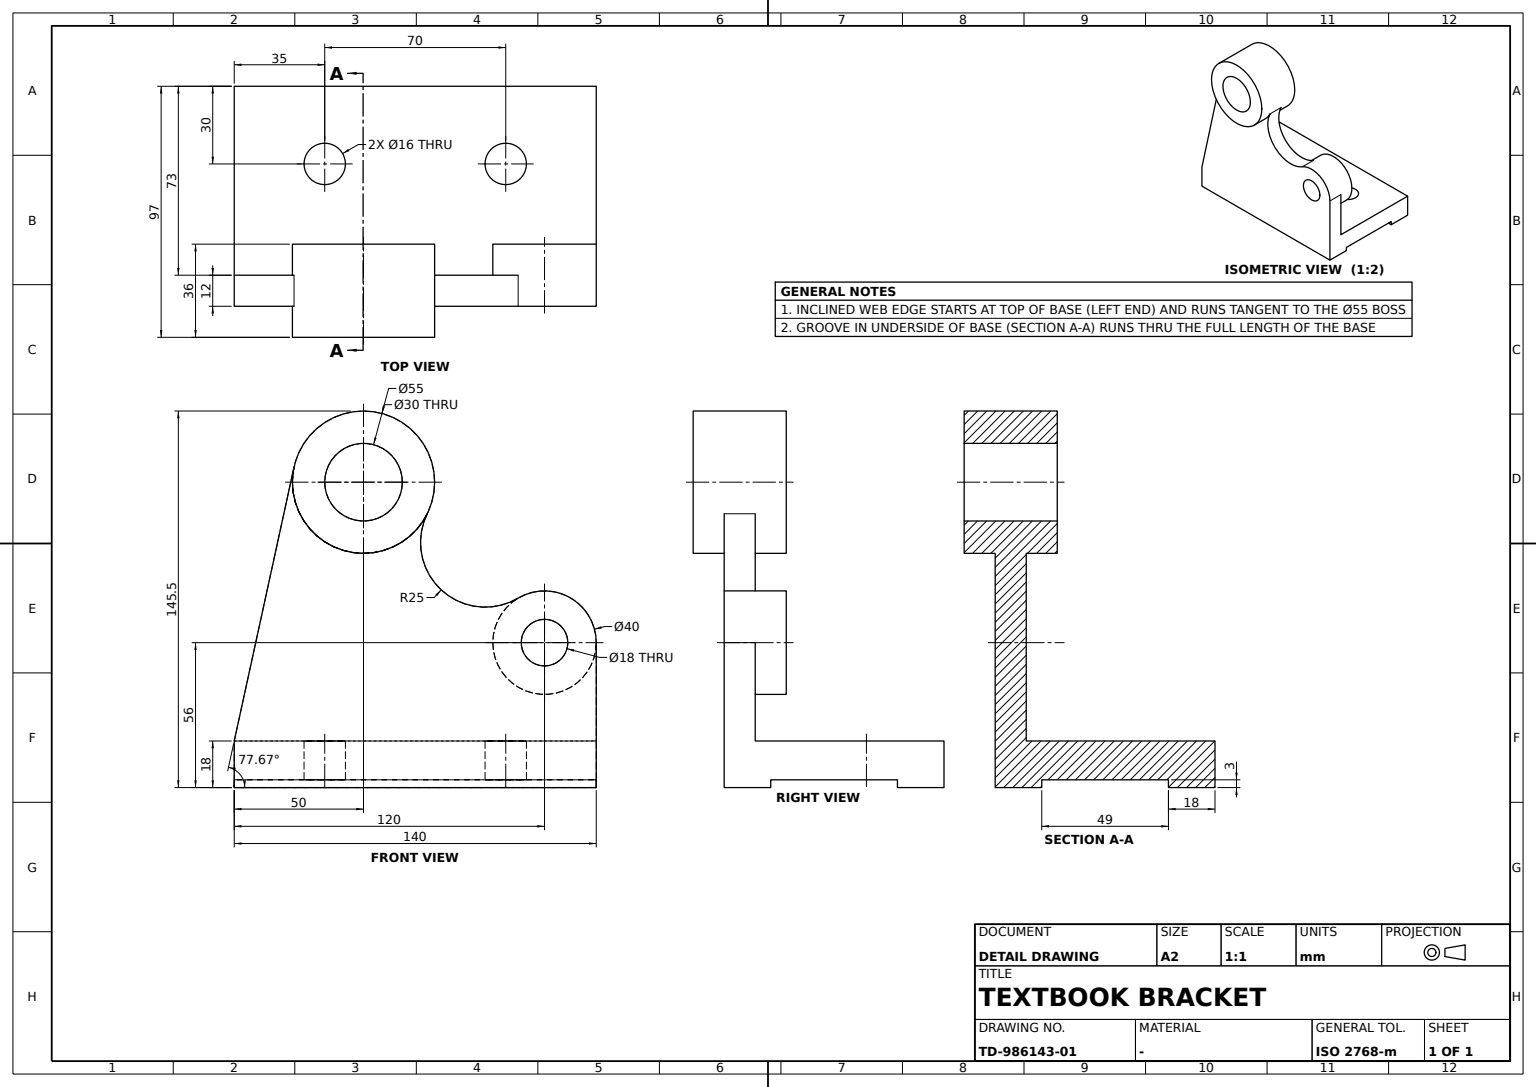
ISO-10303-21;
HEADER;
FILE_DESCRIPTION((''),'2;1');
FILE_NAME('','',(''),(''),'','','');
FILE_SCHEMA(('AUTOMOTIVE_DESIGN'));
ENDSEC;
DATA;
#1=APPLICATION_CONTEXT('');
#2=PRODUCT_CONTEXT('',#1,'mechanical');
#3=PRODUCT('','','',(#2));
#4=PRODUCT_DEFINITION_FORMATION('','',#3);
#5=PRODUCT_DEFINITION_CONTEXT('',#1,'design');
#6=PRODUCT_DEFINITION('','',#4,#5);
#7=PRODUCT_DEFINITION_SHAPE('','',#6);
#8=(LENGTH_UNIT()NAMED_UNIT(*)SI_UNIT(.MILLI.,.METRE.));
#9=(NAMED_UNIT(*)PLANE_ANGLE_UNIT()SI_UNIT($,.RADIAN.));
#10=(NAMED_UNIT(*)SI_UNIT($,.STERADIAN.)SOLID_ANGLE_UNIT());
#11=UNCERTAINTY_MEASURE_WITH_UNIT(LENGTH_MEASURE(1.E-05),#8,'distance_accuracy_value','');
#12=(GEOMETRIC_REPRESENTATION_CONTEXT(3)GLOBAL_UNCERTAINTY_ASSIGNED_CONTEXT((#11))GLOBAL_UNIT_ASSIGNED_CONTEXT((#8,#9,#10))REPRESENTATION_CONTEXT('',''));
#13=CARTESIAN_POINT('',(43.,12.5,0.));
#14=VERTEX_POINT('',#13);
#15=CARTESIAN_POINT('',(43.,12.5,-15.));
#16=VERTEX_POINT('',#15);
#17=CARTESIAN_POINT('',(43.,12.5,-35.));
#18=DIRECTION('',(0.,0.,-1.));
#19=VECTOR('',#18,1000.);
#20=LINE('',#17,#19);
#21=EDGE_CURVE('',#14,#16,#20,.T.);
#22=ORIENTED_EDGE('',*,*,#21,.F.);
#23=CARTESIAN_POINT('',(27.,12.5,0.));
#24=VERTEX_POINT('',#23);
#25=CARTESIAN_POINT('',(35.,12.5,0.));
#26=DIRECTION('',(0.,0.,1.));
#27=DIRECTION('',(1.,0.,0.));
#28=AXIS2_PLACEMENT_3D('',#25,#26,#27);
#29=CIRCLE('',#28,8.);
#30=EDGE_CURVE('',#14,#24,#29,.T.);
#31=ORIENTED_EDGE('',*,*,#30,.T.);
#32=CARTESIAN_POINT('',(27.,12.5,-15.));
#33=VERTEX_POINT('',#32);
#34=CARTESIAN_POINT('',(27.,12.5,-35.));
#35=LINE('',#34,#19);
#36=EDGE_CURVE('',#24,#33,#35,.T.);
#37=ORIENTED_EDGE('',*,*,#36,.T.);
#38=CARTESIAN_POINT('',(35.,12.5,-15.));
#39=DIRECTION('',(0.,1.,0.));
#40=AXIS2_PLACEMENT_3D('',#38,#18,#39);
#41=CIRCLE('',#40,8.);
#42=EDGE_CURVE('',#33,#16,#41,.T.);
#43=ORIENTED_EDGE('',*,*,#42,.T.);
#44=EDGE_LOOP('',(#22,#31,#37,#43));
#45=FACE_OUTER_BOUND('',#44,.T.);
#46=CARTESIAN_POINT('',(35.,12.5,-35.));
#47=AXIS2_PLACEMENT_3D('',#46,#18,#27);
#48=CYLINDRICAL_SURFACE('',#47,8.);
#49=ADVANCED_FACE('',(#45),#48,.F.);
#50=CARTESIAN_POINT('',(70.,-30.5,38.));
#51=VERTEX_POINT('',#50);
#52=CARTESIAN_POINT('',(70.,-18.5,38.));
#53=VERTEX_POINT('',#52);
#54=CARTESIAN_POINT('',(70.,-39.5,38.));
#55=VECTOR('',#39,1000.);
#56=LINE('',#54,#55);
#57=EDGE_CURVE('',#51,#53,#56,.T.);
#58=ORIENTED_EDGE('',*,*,#57,.F.);
#59=CARTESIAN_POINT('',(30.,-30.5,38.));
#60=VERTEX_POINT('',#59);
#61=CARTESIAN_POINT('',(50.,-30.5,38.));
#62=AXIS2_PLACEMENT_3D('',#61,#39,#27);
#63=CIRCLE('',#62,20.);
#64=EDGE_CURVE('',#51,#60,#63,.T.);
#65=ORIENTED_EDGE('',*,*,#64,.T.);
#66=CARTESIAN_POINT('',(30.,-18.5,38.));
#67=VERTEX_POINT('',#66);
#68=CARTESIAN_POINT('',(30.,-39.5,38.));
#69=LINE('',#68,#55);
#70=EDGE_CURVE('',#60,#67,#69,.T.);
#71=ORIENTED_EDGE('',*,*,#70,.T.);
#72=CARTESIAN_POINT('',(50.,-18.5,38.));
#73=DIRECTION('',(0.,-1.,0.));
#74=AXIS2_PLACEMENT_3D('',#72,#73,#27);
#75=CIRCLE('',#74,20.);
#76=EDGE_CURVE('',#67,#53,#75,.T.);
#77=ORIENTED_EDGE('',*,*,#76,.T.);
#78=EDGE_LOOP('',(#58,#65,#71,#77));
#79=FACE_OUTER_BOUND('',#78,.T.);
#80=CYLINDRICAL_SURFACE('',#62,20.);
#81=ADVANCED_FACE('',(#79),#80,.T.);
#82=CARTESIAN_POINT('',(39.8001548126,-30.5,55.2035798063));
#83=VERTEX_POINT('',#82);
#84=EDGE_CURVE('',#60,#83,#63,.T.);
#85=ORIENTED_EDGE('',*,*,#84,.F.);
#86=ORIENTED_EDGE('',*,*,#64,.F.);
#87=CARTESIAN_POINT('',(70.,-30.5,0.));
#88=VERTEX_POINT('',#87);
#89=CARTESIAN_POINT('',(70.,-30.5,19.));
#90=VECTOR('',#26,1000.);
#91=LINE('',#89,#90);
#92=EDGE_CURVE('',#88,#51,#91,.T.);
#93=ORIENTED_EDGE('',*,*,#92,.F.);
#94=CARTESIAN_POINT('',(-70.,-30.5,0.));
#95=VERTEX_POINT('',#94);
#96=CARTESIAN_POINT('',(0.,-30.5,0.));
#97=VECTOR('',#27,1000.);
#98=LINE('',#96,#97);
#99=EDGE_CURVE('',#95,#88,#98,.T.);
#100=ORIENTED_EDGE('',*,*,#99,.F.);
#101=CARTESIAN_POINT('',(-46.8660884819,-30.5,105.8705442409));
#102=VERTEX_POINT('',#101);
#103=CARTESIAN_POINT('',(-58.4330442409,-30.5,52.9352721205));
#104=DIRECTION('',(-0.213474336,0.,-0.9769486721));
#105=VECTOR('',#104,1000.);
#106=LINE('',#103,#105);
#107=EDGE_CURVE('',#102,#95,#106,.T.);
#108=ORIENTED_EDGE('',*,*,#107,.F.);
#109=CARTESIAN_POINT('',(-47.5,-30.5,100.));
#110=VERTEX_POINT('',#109);
#111=CARTESIAN_POINT('',(-20.,-30.5,100.));
#112=AXIS2_PLACEMENT_3D('',#111,#39,#27);
#113=CIRCLE('',#112,27.5);
#114=EDGE_CURVE('',#110,#102,#113,.T.);
#115=ORIENTED_EDGE('',*,*,#114,.F.);
#116=CARTESIAN_POINT('',(4.6454205529,-30.5,87.7994571527));
#117=VERTEX_POINT('',#116);
#118=EDGE_CURVE('',#117,#110,#113,.T.);
#119=ORIENTED_EDGE('',*,*,#118,.F.);
#120=CARTESIAN_POINT('',(27.0503483283,-30.5,76.7080545643));
#121=AXIS2_PLACEMENT_3D('',#120,#39,#27);
#122=CIRCLE('',#121,25.);
#123=EDGE_CURVE('',#83,#117,#122,.T.);
#124=ORIENTED_EDGE('',*,*,#123,.F.);
#125=EDGE_LOOP('',(#85,#86,#93,#100,#108,#115,#119,#124));
#126=FACE_OUTER_BOUND('',#125,.T.);
#127=AXIS2_PLACEMENT_3D('',#96,#73,#27);
#128=PLANE('',#127);
#129=ADVANCED_FACE('',(#126),#128,.F.);
#130=CARTESIAN_POINT('',(-27.,12.5,0.));
#131=VERTEX_POINT('',#130);
#132=CARTESIAN_POINT('',(-27.,12.5,-15.));
#133=VERTEX_POINT('',#132);
#134=CARTESIAN_POINT('',(-27.,12.5,-35.));
#135=LINE('',#134,#19);
#136=EDGE_CURVE('',#131,#133,#135,.T.);
#137=ORIENTED_EDGE('',*,*,#136,.T.);
#138=CARTESIAN_POINT('',(-43.,12.5,-15.));
#139=VERTEX_POINT('',#138);
#140=CARTESIAN_POINT('',(-35.,12.5,-15.));
#141=AXIS2_PLACEMENT_3D('',#140,#18,#39);
#142=CIRCLE('',#141,8.);
#143=EDGE_CURVE('',#133,#139,#142,.T.);
#144=ORIENTED_EDGE('',*,*,#143,.T.);
#145=CARTESIAN_POINT('',(-43.,12.5,0.));
#146=VERTEX_POINT('',#145);
#147=CARTESIAN_POINT('',(-43.,12.5,-35.));
#148=LINE('',#147,#19);
#149=EDGE_CURVE('',#146,#139,#148,.T.);
#150=ORIENTED_EDGE('',*,*,#149,.F.);
#151=CARTESIAN_POINT('',(-35.,12.5,0.));
#152=AXIS2_PLACEMENT_3D('',#151,#26,#27);
#153=CIRCLE('',#152,8.);
#154=EDGE_CURVE('',#146,#131,#153,.T.);
#155=ORIENTED_EDGE('',*,*,#154,.T.);
#156=EDGE_LOOP('',(#137,#144,#150,#155));
#157=FACE_OUTER_BOUND('',#156,.T.);
#158=CARTESIAN_POINT('',(-35.,12.5,-35.));
#159=AXIS2_PLACEMENT_3D('',#158,#18,#27);
#160=CYLINDRICAL_SURFACE('',#159,8.);
#161=ADVANCED_FACE('',(#157),#160,.F.);
#162=CARTESIAN_POINT('',(59.,-18.5,38.));
#163=VERTEX_POINT('',#162);
#164=CARTESIAN_POINT('',(41.,-18.5,38.));
#165=VERTEX_POINT('',#164);
#166=DIRECTION('',(-1.,0.,0.));
#167=AXIS2_PLACEMENT_3D('',#72,#39,#166);
#168=CIRCLE('',#167,9.);
#169=EDGE_CURVE('',#163,#165,#168,.T.);
#170=ORIENTED_EDGE('',*,*,#169,.T.);
#171=CARTESIAN_POINT('',(41.,-42.5,38.));
#172=VERTEX_POINT('',#171);
#173=CARTESIAN_POINT('',(41.,-30.5,38.));
#174=VECTOR('',#73,1000.);
#175=LINE('',#173,#174);
#176=EDGE_CURVE('',#165,#172,#175,.T.);
#177=ORIENTED_EDGE('',*,*,#176,.T.);
#178=CARTESIAN_POINT('',(59.,-42.5,38.));
#179=VERTEX_POINT('',#178);
#180=CARTESIAN_POINT('',(50.,-42.5,38.));
#181=AXIS2_PLACEMENT_3D('',#180,#39,#166);
#182=CIRCLE('',#181,9.);
#183=EDGE_CURVE('',#179,#172,#182,.T.);
#184=ORIENTED_EDGE('',*,*,#183,.F.);
#185=CARTESIAN_POINT('',(59.,-30.5,38.));
#186=LINE('',#185,#174);
#187=EDGE_CURVE('',#163,#179,#186,.T.);
#188=ORIENTED_EDGE('',*,*,#187,.F.);
#189=EDGE_LOOP('',(#170,#177,#184,#188));
#190=FACE_OUTER_BOUND('',#189,.T.);
#191=AXIS2_PLACEMENT_3D('',#61,#73,#166);
#192=CYLINDRICAL_SURFACE('',#191,9.);
#193=ADVANCED_FACE('',(#190),#192,.F.);
#194=CARTESIAN_POINT('',(39.8001548126,-42.5,55.2035798063));
#195=VERTEX_POINT('',#194);
#196=CARTESIAN_POINT('',(4.6454205529,-42.5,87.7994571527));
#197=VERTEX_POINT('',#196);
#198=CARTESIAN_POINT('',(27.0503483283,-42.5,76.7080545643));
#199=AXIS2_PLACEMENT_3D('',#198,#39,#27);
#200=CIRCLE('',#199,25.);
#201=EDGE_CURVE('',#195,#197,#200,.T.);
#202=ORIENTED_EDGE('',*,*,#201,.F.);
#203=CARTESIAN_POINT('',(39.8001548126,-39.5,55.2035798063));
#204=LINE('',#203,#55);
#205=EDGE_CURVE('',#195,#83,#204,.T.);
#206=ORIENTED_EDGE('',*,*,#205,.T.);
#207=ORIENTED_EDGE('',*,*,#123,.T.);
#208=CARTESIAN_POINT('',(4.6454205529,-36.5,87.7994571527));
#209=LINE('',#208,#55);
#210=EDGE_CURVE('',#197,#117,#209,.T.);
#211=ORIENTED_EDGE('',*,*,#210,.F.);
#212=EDGE_LOOP('',(#202,#206,#207,#211));
#213=FACE_OUTER_BOUND('',#212,.T.);
#214=CARTESIAN_POINT('',(27.0503483283,-36.5,76.7080545643));
#215=AXIS2_PLACEMENT_3D('',#214,#39,#27);
#216=CYLINDRICAL_SURFACE('',#215,25.);
#217=ADVANCED_FACE('',(#213),#216,.F.);
#218=CARTESIAN_POINT('',(-70.,24.5,-18.));
#219=VERTEX_POINT('',#218);
#220=CARTESIAN_POINT('',(70.,24.5,-18.));
#221=VERTEX_POINT('',#220);
#222=CARTESIAN_POINT('',(0.,24.5,-18.));
#223=LINE('',#222,#97);
#224=EDGE_CURVE('',#219,#221,#223,.T.);
#225=ORIENTED_EDGE('',*,*,#224,.F.);
#226=CARTESIAN_POINT('',(-70.,42.5,-18.));
#227=VERTEX_POINT('',#226);
#228=CARTESIAN_POINT('',(-70.,33.5,-18.));
#229=LINE('',#228,#55);
#230=EDGE_CURVE('',#219,#227,#229,.T.);
#231=ORIENTED_EDGE('',*,*,#230,.T.);
#232=CARTESIAN_POINT('',(70.,42.5,-18.));
#233=VERTEX_POINT('',#232);
#234=CARTESIAN_POINT('',(0.,42.5,-18.));
#235=LINE('',#234,#97);
#236=EDGE_CURVE('',#227,#233,#235,.T.);
#237=ORIENTED_EDGE('',*,*,#236,.T.);
#238=CARTESIAN_POINT('',(70.,33.5,-18.));
#239=LINE('',#238,#55);
#240=EDGE_CURVE('',#221,#233,#239,.T.);
#241=ORIENTED_EDGE('',*,*,#240,.F.);
#242=EDGE_LOOP('',(#225,#231,#237,#241));
#243=FACE_OUTER_BOUND('',#242,.T.);
#244=CARTESIAN_POINT('',(0.,-42.5,-18.));
#245=AXIS2_PLACEMENT_3D('',#244,#18,#39);
#246=PLANE('',#245);
#247=ADVANCED_FACE('',(#243),#246,.T.);
#248=CARTESIAN_POINT('',(-47.5,-18.5,100.));
#249=VERTEX_POINT('',#248);
#250=CARTESIAN_POINT('',(-47.5,-39.5,100.));
#251=LINE('',#250,#174);
#252=EDGE_CURVE('',#249,#110,#251,.T.);
#253=ORIENTED_EDGE('',*,*,#252,.F.);
#254=CARTESIAN_POINT('',(7.5,-18.5,100.));
#255=VERTEX_POINT('',#254);
#256=CARTESIAN_POINT('',(-20.,-18.5,100.));
#257=AXIS2_PLACEMENT_3D('',#256,#73,#27);
#258=CIRCLE('',#257,27.5);
#259=EDGE_CURVE('',#249,#255,#258,.T.);
#260=ORIENTED_EDGE('',*,*,#259,.T.);
#261=CARTESIAN_POINT('',(7.5,-54.5,100.));
#262=VERTEX_POINT('',#261);
#263=CARTESIAN_POINT('',(7.5,-39.5,100.));
#264=LINE('',#263,#174);
#265=EDGE_CURVE('',#255,#262,#264,.T.);
#266=ORIENTED_EDGE('',*,*,#265,.T.);
#267=CARTESIAN_POINT('',(-47.5,-54.5,100.));
#268=VERTEX_POINT('',#267);
#269=CARTESIAN_POINT('',(-20.,-54.5,100.));
#270=AXIS2_PLACEMENT_3D('',#269,#73,#27);
#271=CIRCLE('',#270,27.5);
#272=EDGE_CURVE('',#268,#262,#271,.T.);
#273=ORIENTED_EDGE('',*,*,#272,.F.);
#274=CARTESIAN_POINT('',(-47.5,-42.5,100.));
#275=VERTEX_POINT('',#274);
#276=EDGE_CURVE('',#275,#268,#251,.T.);
#277=ORIENTED_EDGE('',*,*,#276,.F.);
#278=CARTESIAN_POINT('',(-20.,-42.5,100.));
#279=AXIS2_PLACEMENT_3D('',#278,#39,#27);
#280=CIRCLE('',#279,27.5);
#281=EDGE_CURVE('',#197,#275,#280,.T.);
#282=ORIENTED_EDGE('',*,*,#281,.F.);
#283=ORIENTED_EDGE('',*,*,#210,.T.);
#284=ORIENTED_EDGE('',*,*,#118,.T.);
#285=EDGE_LOOP('',(#253,#260,#266,#273,#277,#282,#283,#284));
#286=FACE_OUTER_BOUND('',#285,.T.);
#287=CARTESIAN_POINT('',(-20.,-36.5,100.));
#288=AXIS2_PLACEMENT_3D('',#287,#39,#27);
#289=CYLINDRICAL_SURFACE('',#288,27.5);
#290=ADVANCED_FACE('',(#286),#289,.T.);
#291=CARTESIAN_POINT('',(-70.,-42.5,0.));
#292=VERTEX_POINT('',#291);
#293=CARTESIAN_POINT('',(-70.,-36.5,0.));
#294=LINE('',#293,#174);
#295=EDGE_CURVE('',#95,#292,#294,.T.);
#296=ORIENTED_EDGE('',*,*,#295,.T.);
#297=CARTESIAN_POINT('',(-46.8660884819,-42.5,105.8705442409));
#298=VERTEX_POINT('',#297);
#299=CARTESIAN_POINT('',(-58.4330442409,-42.5,52.9352721205));
#300=LINE('',#299,#105);
#301=EDGE_CURVE('',#298,#292,#300,.T.);
#302=ORIENTED_EDGE('',*,*,#301,.F.);
#303=CARTESIAN_POINT('',(-46.8660884819,-39.5,105.8705442409));
#304=LINE('',#303,#55);
#305=EDGE_CURVE('',#298,#102,#304,.T.);
#306=ORIENTED_EDGE('',*,*,#305,.T.);
#307=ORIENTED_EDGE('',*,*,#107,.T.);
#308=EDGE_LOOP('',(#296,#302,#306,#307));
#309=FACE_OUTER_BOUND('',#308,.T.);
#310=DIRECTION('',(-0.9769486721,0.,0.213474336));
#311=DIRECTION('',(0.213474336,0.,0.9769486721));
#312=AXIS2_PLACEMENT_3D('',#291,#310,#311);
#313=PLANE('',#312);
#314=ADVANCED_FACE('',(#309),#313,.T.);
#315=CARTESIAN_POINT('',(-35.,-18.5,100.));
#316=VERTEX_POINT('',#315);
#317=CARTESIAN_POINT('',(-35.,-54.5,100.));
#318=VERTEX_POINT('',#317);
#319=CARTESIAN_POINT('',(-35.,-37.1600000005,100.));
#320=LINE('',#319,#174);
#321=EDGE_CURVE('',#316,#318,#320,.T.);
#322=ORIENTED_EDGE('',*,*,#321,.F.);
#323=CARTESIAN_POINT('',(-5.,-18.5,100.));
#324=VERTEX_POINT('',#323);
#325=AXIS2_PLACEMENT_3D('',#256,#39,#166);
#326=CIRCLE('',#325,15.);
#327=EDGE_CURVE('',#316,#324,#326,.T.);
#328=ORIENTED_EDGE('',*,*,#327,.T.);
#329=CARTESIAN_POINT('',(-5.,-54.5,100.));
#330=VERTEX_POINT('',#329);
#331=CARTESIAN_POINT('',(-5.,-37.1600000005,100.));
#332=LINE('',#331,#174);
#333=EDGE_CURVE('',#324,#330,#332,.T.);
#334=ORIENTED_EDGE('',*,*,#333,.T.);
#335=CIRCLE('',#270,15.);
#336=EDGE_CURVE('',#330,#318,#335,.T.);
#337=ORIENTED_EDGE('',*,*,#336,.T.);
#338=EDGE_LOOP('',(#322,#328,#334,#337));
#339=FACE_OUTER_BOUND('',#338,.T.);
#340=CARTESIAN_POINT('',(-20.,-37.1600000005,100.));
#341=AXIS2_PLACEMENT_3D('',#340,#73,#166);
#342=CYLINDRICAL_SURFACE('',#341,15.);
#343=ADVANCED_FACE('',(#339),#342,.F.);
#344=ORIENTED_EDGE('',*,*,#21,.T.);
#345=EDGE_CURVE('',#16,#33,#41,.T.);
#346=ORIENTED_EDGE('',*,*,#345,.T.);
#347=ORIENTED_EDGE('',*,*,#36,.F.);
#348=EDGE_CURVE('',#24,#14,#29,.T.);
#349=ORIENTED_EDGE('',*,*,#348,.T.);
#350=EDGE_LOOP('',(#344,#346,#347,#349));
#351=FACE_OUTER_BOUND('',#350,.T.);
#352=ADVANCED_FACE('',(#351),#48,.F.);
#353=CARTESIAN_POINT('',(-70.,42.5,0.));
#354=VERTEX_POINT('',#353);
#355=CARTESIAN_POINT('',(-70.,6.,0.));
#356=LINE('',#355,#174);
#357=EDGE_CURVE('',#354,#95,#356,.T.);
#358=ORIENTED_EDGE('',*,*,#357,.T.);
#359=ORIENTED_EDGE('',*,*,#99,.T.);
#360=CARTESIAN_POINT('',(70.,42.5,0.));
#361=VERTEX_POINT('',#360);
#362=CARTESIAN_POINT('',(70.,6.,0.));
#363=LINE('',#362,#174);
#364=EDGE_CURVE('',#361,#88,#363,.T.);
#365=ORIENTED_EDGE('',*,*,#364,.F.);
#366=CARTESIAN_POINT('',(0.,42.5,0.));
#367=LINE('',#366,#97);
#368=EDGE_CURVE('',#354,#361,#367,.T.);
#369=ORIENTED_EDGE('',*,*,#368,.F.);
#370=EDGE_LOOP('',(#358,#359,#365,#369));
#371=FACE_OUTER_BOUND('',#370,.T.);
#372=ORIENTED_EDGE('',*,*,#30,.F.);
#373=ORIENTED_EDGE('',*,*,#348,.F.);
#374=EDGE_LOOP('',(#372,#373));
#375=FACE_BOUND('',#374,.T.);
#376=ORIENTED_EDGE('',*,*,#154,.F.);
#377=EDGE_CURVE('',#131,#146,#153,.T.);
#378=ORIENTED_EDGE('',*,*,#377,.F.);
#379=EDGE_LOOP('',(#376,#378));
#380=FACE_BOUND('',#379,.T.);
#381=CARTESIAN_POINT('',(0.,-42.5,0.));
#382=AXIS2_PLACEMENT_3D('',#381,#18,#39);
#383=PLANE('',#382);
#384=ADVANCED_FACE('',(#371,#375,#380),#383,.F.);
#385=CARTESIAN_POINT('',(-70.,-42.5,-18.));
#386=VERTEX_POINT('',#385);
#387=CARTESIAN_POINT('',(-70.,-24.5,-18.));
#388=VERTEX_POINT('',#387);
#389=CARTESIAN_POINT('',(-70.,-33.5,-18.));
#390=LINE('',#389,#55);
#391=EDGE_CURVE('',#386,#388,#390,.T.);
#392=ORIENTED_EDGE('',*,*,#391,.T.);
#393=CARTESIAN_POINT('',(70.,-24.5,-18.));
#394=VERTEX_POINT('',#393);
#395=CARTESIAN_POINT('',(0.,-24.5,-18.));
#396=LINE('',#395,#97);
#397=EDGE_CURVE('',#388,#394,#396,.T.);
#398=ORIENTED_EDGE('',*,*,#397,.T.);
#399=CARTESIAN_POINT('',(70.,-42.5,-18.));
#400=VERTEX_POINT('',#399);
#401=CARTESIAN_POINT('',(70.,-33.5,-18.));
#402=LINE('',#401,#55);
#403=EDGE_CURVE('',#400,#394,#402,.T.);
#404=ORIENTED_EDGE('',*,*,#403,.F.);
#405=LINE('',#244,#97);
#406=EDGE_CURVE('',#386,#400,#405,.T.);
#407=ORIENTED_EDGE('',*,*,#406,.F.);
#408=EDGE_LOOP('',(#392,#398,#404,#407));
#409=FACE_OUTER_BOUND('',#408,.T.);
#410=ADVANCED_FACE('',(#409),#246,.T.);
#411=EDGE_CURVE('',#53,#67,#75,.T.);
#412=ORIENTED_EDGE('',*,*,#411,.F.);
#413=ORIENTED_EDGE('',*,*,#76,.F.);
#414=EDGE_LOOP('',(#412,#413));
#415=FACE_OUTER_BOUND('',#414,.T.);
#416=EDGE_CURVE('',#165,#163,#168,.T.);
#417=ORIENTED_EDGE('',*,*,#416,.F.);
#418=ORIENTED_EDGE('',*,*,#169,.F.);
#419=EDGE_LOOP('',(#417,#418));
#420=FACE_BOUND('',#419,.T.);
#421=CARTESIAN_POINT('',(0.,-18.5,0.));
#422=AXIS2_PLACEMENT_3D('',#421,#73,#27);
#423=PLANE('',#422);
#424=ADVANCED_FACE('',(#415,#420),#423,.F.);
#425=ORIENTED_EDGE('',*,*,#327,.F.);
#426=EDGE_CURVE('',#324,#316,#326,.T.);
#427=ORIENTED_EDGE('',*,*,#426,.F.);
#428=EDGE_LOOP('',(#425,#427));
#429=FACE_BOUND('',#428,.T.);
#430=ORIENTED_EDGE('',*,*,#259,.F.);
#431=EDGE_CURVE('',#255,#249,#258,.T.);
#432=ORIENTED_EDGE('',*,*,#431,.F.);
#433=EDGE_LOOP('',(#430,#432));
#434=FACE_OUTER_BOUND('',#433,.T.);
#435=ADVANCED_FACE('',(#429,#434),#423,.F.);
#436=ORIENTED_EDGE('',*,*,#272,.T.);
#437=EDGE_CURVE('',#262,#268,#271,.T.);
#438=ORIENTED_EDGE('',*,*,#437,.T.);
#439=EDGE_LOOP('',(#436,#438));
#440=FACE_OUTER_BOUND('',#439,.T.);
#441=ORIENTED_EDGE('',*,*,#336,.F.);
#442=EDGE_CURVE('',#318,#330,#335,.T.);
#443=ORIENTED_EDGE('',*,*,#442,.F.);
#444=EDGE_LOOP('',(#441,#443));
#445=FACE_BOUND('',#444,.T.);
#446=CARTESIAN_POINT('',(0.,-54.5,0.));
#447=AXIS2_PLACEMENT_3D('',#446,#73,#27);
#448=PLANE('',#447);
#449=ADVANCED_FACE('',(#440,#445),#448,.T.);
#450=ORIENTED_EDGE('',*,*,#201,.T.);
#451=ORIENTED_EDGE('',*,*,#281,.T.);
#452=EDGE_CURVE('',#275,#298,#280,.T.);
#453=ORIENTED_EDGE('',*,*,#452,.T.);
#454=ORIENTED_EDGE('',*,*,#301,.T.);
#455=CARTESIAN_POINT('',(-70.,-42.5,-9.));
#456=LINE('',#455,#19);
#457=EDGE_CURVE('',#292,#386,#456,.T.);
#458=ORIENTED_EDGE('',*,*,#457,.T.);
#459=ORIENTED_EDGE('',*,*,#406,.T.);
#460=CARTESIAN_POINT('',(70.,-42.5,38.));
#461=VERTEX_POINT('',#460);
#462=CARTESIAN_POINT('',(70.,-42.5,10.));
#463=LINE('',#462,#19);
#464=EDGE_CURVE('',#461,#400,#463,.T.);
#465=ORIENTED_EDGE('',*,*,#464,.F.);
#466=AXIS2_PLACEMENT_3D('',#180,#73,#27);
#467=CIRCLE('',#466,20.);
#468=EDGE_CURVE('',#461,#195,#467,.T.);
#469=ORIENTED_EDGE('',*,*,#468,.T.);
#470=EDGE_LOOP('',(#450,#451,#453,#454,#458,#459,#465,#469));
#471=FACE_OUTER_BOUND('',#470,.T.);
#472=EDGE_CURVE('',#172,#179,#182,.T.);
#473=ORIENTED_EDGE('',*,*,#472,.T.);
#474=ORIENTED_EDGE('',*,*,#183,.T.);
#475=EDGE_LOOP('',(#473,#474));
#476=FACE_BOUND('',#475,.T.);
#477=AXIS2_PLACEMENT_3D('',#381,#73,#18);
#478=PLANE('',#477);
#479=ADVANCED_FACE('',(#471,#476),#478,.T.);
#480=CARTESIAN_POINT('',(70.,-36.5,38.));
#481=LINE('',#480,#55);
#482=EDGE_CURVE('',#461,#51,#481,.T.);
#483=ORIENTED_EDGE('',*,*,#482,.F.);
#484=ORIENTED_EDGE('',*,*,#464,.T.);
#485=ORIENTED_EDGE('',*,*,#403,.T.);
#486=CARTESIAN_POINT('',(70.,-24.5,-15.));
#487=VERTEX_POINT('',#486);
#488=CARTESIAN_POINT('',(70.,-24.5,-16.5));
#489=LINE('',#488,#90);
#490=EDGE_CURVE('',#394,#487,#489,.T.);
#491=ORIENTED_EDGE('',*,*,#490,.T.);
#492=CARTESIAN_POINT('',(70.,24.5,-15.));
#493=VERTEX_POINT('',#492);
#494=CARTESIAN_POINT('',(70.,0.,-15.));
#495=LINE('',#494,#55);
#496=EDGE_CURVE('',#487,#493,#495,.T.);
#497=ORIENTED_EDGE('',*,*,#496,.T.);
#498=CARTESIAN_POINT('',(70.,24.5,-16.5));
#499=LINE('',#498,#19);
#500=EDGE_CURVE('',#493,#221,#499,.T.);
#501=ORIENTED_EDGE('',*,*,#500,.T.);
#502=ORIENTED_EDGE('',*,*,#240,.T.);
#503=CARTESIAN_POINT('',(70.,42.5,-9.));
#504=LINE('',#503,#90);
#505=EDGE_CURVE('',#233,#361,#504,.T.);
#506=ORIENTED_EDGE('',*,*,#505,.T.);
#507=ORIENTED_EDGE('',*,*,#364,.T.);
#508=ORIENTED_EDGE('',*,*,#92,.T.);
#509=EDGE_LOOP('',(#483,#484,#485,#491,#497,#501,#502,#506,#507,#508));
#510=FACE_OUTER_BOUND('',#509,.T.);
#511=CARTESIAN_POINT('',(70.,0.,0.));
#512=AXIS2_PLACEMENT_3D('',#511,#27,#39);
#513=PLANE('',#512);
#514=ADVANCED_FACE('',(#510),#513,.T.);
#515=ORIENTED_EDGE('',*,*,#505,.F.);
#516=ORIENTED_EDGE('',*,*,#236,.F.);
#517=CARTESIAN_POINT('',(-70.,42.5,-9.));
#518=LINE('',#517,#90);
#519=EDGE_CURVE('',#227,#354,#518,.T.);
#520=ORIENTED_EDGE('',*,*,#519,.T.);
#521=ORIENTED_EDGE('',*,*,#368,.T.);
#522=EDGE_LOOP('',(#515,#516,#520,#521));
#523=FACE_OUTER_BOUND('',#522,.T.);
#524=AXIS2_PLACEMENT_3D('',#366,#73,#18);
#525=PLANE('',#524);
#526=ADVANCED_FACE('',(#523),#525,.F.);
#527=ORIENTED_EDGE('',*,*,#187,.T.);
#528=ORIENTED_EDGE('',*,*,#472,.F.);
#529=ORIENTED_EDGE('',*,*,#176,.F.);
#530=ORIENTED_EDGE('',*,*,#416,.T.);
#531=EDGE_LOOP('',(#527,#528,#529,#530));
#532=FACE_OUTER_BOUND('',#531,.T.);
#533=ADVANCED_FACE('',(#532),#192,.F.);
#534=ORIENTED_EDGE('',*,*,#411,.T.);
#535=ORIENTED_EDGE('',*,*,#70,.F.);
#536=ORIENTED_EDGE('',*,*,#84,.T.);
#537=ORIENTED_EDGE('',*,*,#205,.F.);
#538=ORIENTED_EDGE('',*,*,#468,.F.);
#539=ORIENTED_EDGE('',*,*,#482,.T.);
#540=ORIENTED_EDGE('',*,*,#57,.T.);
#541=EDGE_LOOP('',(#534,#535,#536,#537,#538,#539,#540));
#542=FACE_OUTER_BOUND('',#541,.T.);
#543=ADVANCED_FACE('',(#542),#80,.T.);
#544=ORIENTED_EDGE('',*,*,#276,.T.);
#545=ORIENTED_EDGE('',*,*,#437,.F.);
#546=ORIENTED_EDGE('',*,*,#265,.F.);
#547=ORIENTED_EDGE('',*,*,#431,.T.);
#548=ORIENTED_EDGE('',*,*,#252,.T.);
#549=ORIENTED_EDGE('',*,*,#114,.T.);
#550=ORIENTED_EDGE('',*,*,#305,.F.);
#551=ORIENTED_EDGE('',*,*,#452,.F.);
#552=EDGE_LOOP('',(#544,#545,#546,#547,#548,#549,#550,#551));
#553=FACE_OUTER_BOUND('',#552,.T.);
#554=ADVANCED_FACE('',(#553),#289,.T.);
#555=ORIENTED_EDGE('',*,*,#295,.F.);
#556=ORIENTED_EDGE('',*,*,#357,.F.);
#557=ORIENTED_EDGE('',*,*,#519,.F.);
#558=ORIENTED_EDGE('',*,*,#230,.F.);
#559=CARTESIAN_POINT('',(-70.,24.5,-15.));
#560=VERTEX_POINT('',#559);
#561=CARTESIAN_POINT('',(-70.,24.5,-16.5));
#562=LINE('',#561,#19);
#563=EDGE_CURVE('',#560,#219,#562,.T.);
#564=ORIENTED_EDGE('',*,*,#563,.F.);
#565=CARTESIAN_POINT('',(-70.,-24.5,-15.));
#566=VERTEX_POINT('',#565);
#567=CARTESIAN_POINT('',(-70.,0.,-15.));
#568=LINE('',#567,#55);
#569=EDGE_CURVE('',#566,#560,#568,.T.);
#570=ORIENTED_EDGE('',*,*,#569,.F.);
#571=CARTESIAN_POINT('',(-70.,-24.5,-16.5));
#572=LINE('',#571,#90);
#573=EDGE_CURVE('',#388,#566,#572,.T.);
#574=ORIENTED_EDGE('',*,*,#573,.F.);
#575=ORIENTED_EDGE('',*,*,#391,.F.);
#576=ORIENTED_EDGE('',*,*,#457,.F.);
#577=EDGE_LOOP('',(#555,#556,#557,#558,#564,#570,#574,#575,#576));
#578=FACE_OUTER_BOUND('',#577,.T.);
#579=CARTESIAN_POINT('',(-70.,0.,0.));
#580=AXIS2_PLACEMENT_3D('',#579,#27,#39);
#581=PLANE('',#580);
#582=ADVANCED_FACE('',(#578),#581,.F.);
#583=ORIENTED_EDGE('',*,*,#573,.T.);
#584=CARTESIAN_POINT('',(0.,-24.5,-15.));
#585=LINE('',#584,#97);
#586=EDGE_CURVE('',#566,#487,#585,.T.);
#587=ORIENTED_EDGE('',*,*,#586,.T.);
#588=ORIENTED_EDGE('',*,*,#490,.F.);
#589=ORIENTED_EDGE('',*,*,#397,.F.);
#590=EDGE_LOOP('',(#583,#587,#588,#589));
#591=FACE_OUTER_BOUND('',#590,.T.);
#592=AXIS2_PLACEMENT_3D('',#395,#39,#26);
#593=PLANE('',#592);
#594=ADVANCED_FACE('',(#591),#593,.T.);
#595=ORIENTED_EDGE('',*,*,#149,.T.);
#596=EDGE_CURVE('',#139,#133,#142,.T.);
#597=ORIENTED_EDGE('',*,*,#596,.T.);
#598=ORIENTED_EDGE('',*,*,#136,.F.);
#599=ORIENTED_EDGE('',*,*,#377,.T.);
#600=EDGE_LOOP('',(#595,#597,#598,#599));
#601=FACE_OUTER_BOUND('',#600,.T.);
#602=ADVANCED_FACE('',(#601),#160,.F.);
#603=ORIENTED_EDGE('',*,*,#563,.T.);
#604=ORIENTED_EDGE('',*,*,#224,.T.);
#605=ORIENTED_EDGE('',*,*,#500,.F.);
#606=CARTESIAN_POINT('',(0.,24.5,-15.));
#607=LINE('',#606,#97);
#608=EDGE_CURVE('',#560,#493,#607,.T.);
#609=ORIENTED_EDGE('',*,*,#608,.F.);
#610=EDGE_LOOP('',(#603,#604,#605,#609));
#611=FACE_OUTER_BOUND('',#610,.T.);
#612=AXIS2_PLACEMENT_3D('',#606,#73,#18);
#613=PLANE('',#612);
#614=ADVANCED_FACE('',(#611),#613,.T.);
#615=ORIENTED_EDGE('',*,*,#569,.T.);
#616=ORIENTED_EDGE('',*,*,#608,.T.);
#617=ORIENTED_EDGE('',*,*,#496,.F.);
#618=ORIENTED_EDGE('',*,*,#586,.F.);
#619=EDGE_LOOP('',(#615,#616,#617,#618));
#620=FACE_OUTER_BOUND('',#619,.T.);
#621=ORIENTED_EDGE('',*,*,#143,.F.);
#622=ORIENTED_EDGE('',*,*,#596,.F.);
#623=EDGE_LOOP('',(#621,#622));
#624=FACE_BOUND('',#623,.T.);
#625=ORIENTED_EDGE('',*,*,#42,.F.);
#626=ORIENTED_EDGE('',*,*,#345,.F.);
#627=EDGE_LOOP('',(#625,#626));
#628=FACE_BOUND('',#627,.T.);
#629=AXIS2_PLACEMENT_3D('',#584,#18,#39);
#630=PLANE('',#629);
#631=ADVANCED_FACE('',(#620,#624,#628),#630,.T.);
#632=ORIENTED_EDGE('',*,*,#333,.F.);
#633=ORIENTED_EDGE('',*,*,#426,.T.);
#634=ORIENTED_EDGE('',*,*,#321,.T.);
#635=ORIENTED_EDGE('',*,*,#442,.T.);
#636=EDGE_LOOP('',(#632,#633,#634,#635));
#637=FACE_OUTER_BOUND('',#636,.T.);
#638=ADVANCED_FACE('',(#637),#342,.F.);
#639=CLOSED_SHELL('',(#49,#81,#129,#161,#193,#217,#247,#290,#314,#343,#352,#384,#410,#424,#435,#449,#479,#514,#526,#533,#543,#554,#582,#594,#602,#614,#631,#638));
#640=MANIFOLD_SOLID_BREP('',#639);
#641=ADVANCED_BREP_SHAPE_REPRESENTATION('',(#640),#12);
#642=SHAPE_DEFINITION_REPRESENTATION(#7,#641);
ENDSEC;
END-ISO-10303-21;
